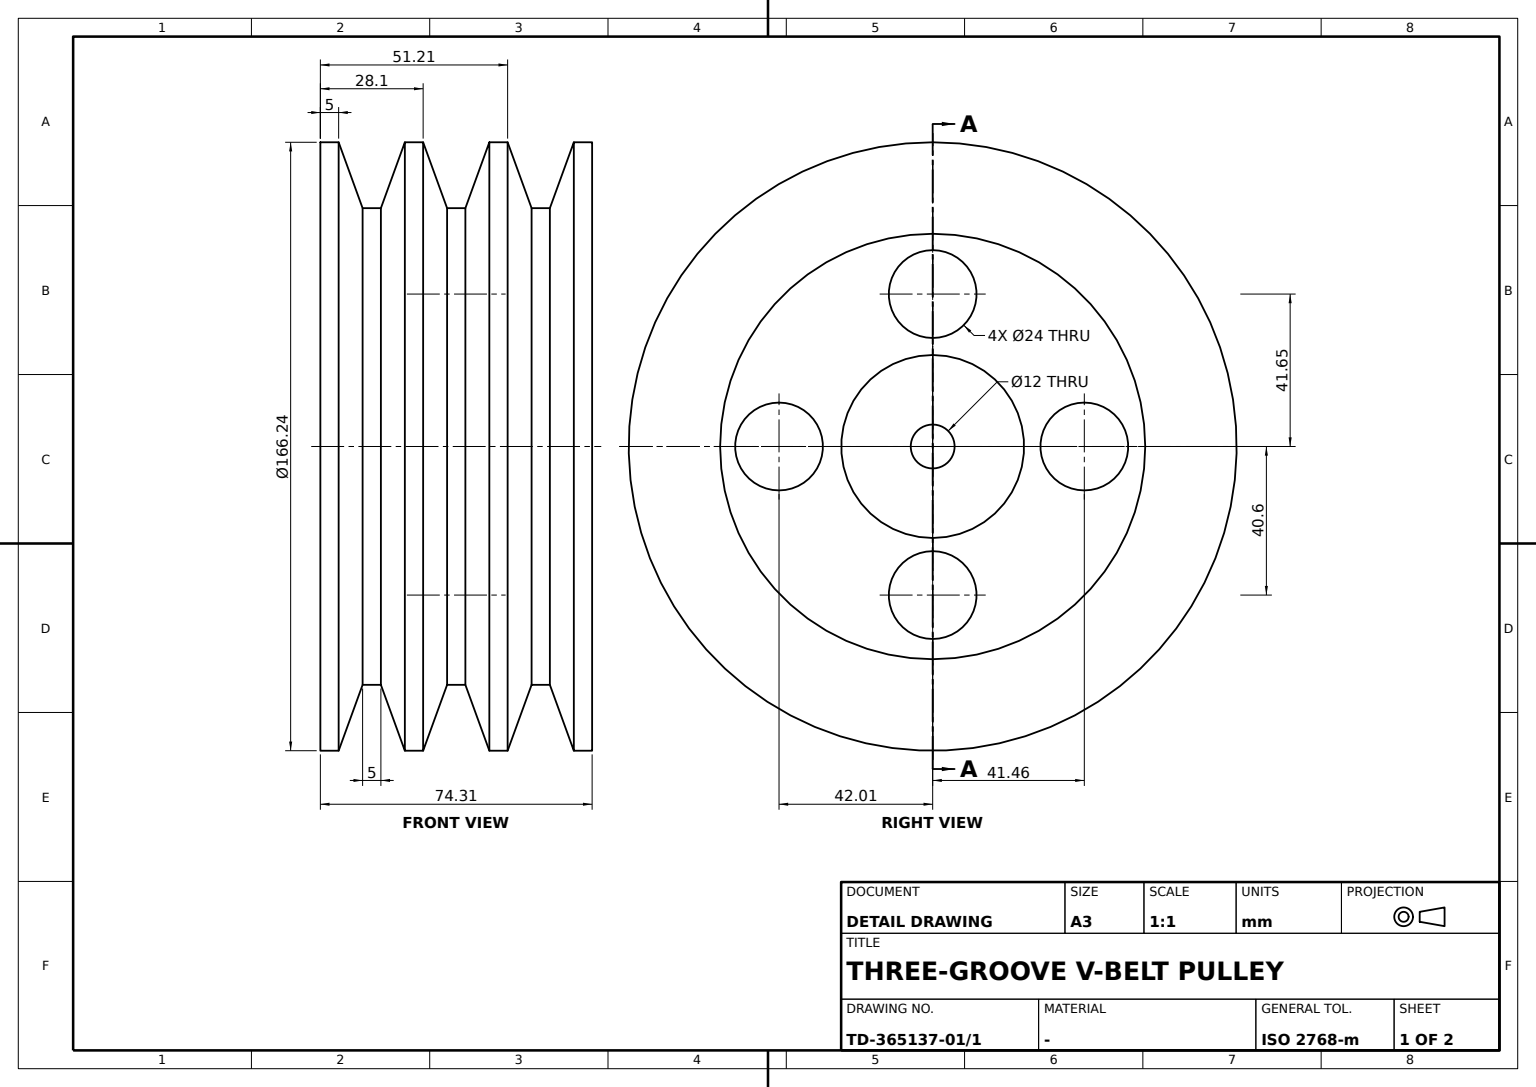
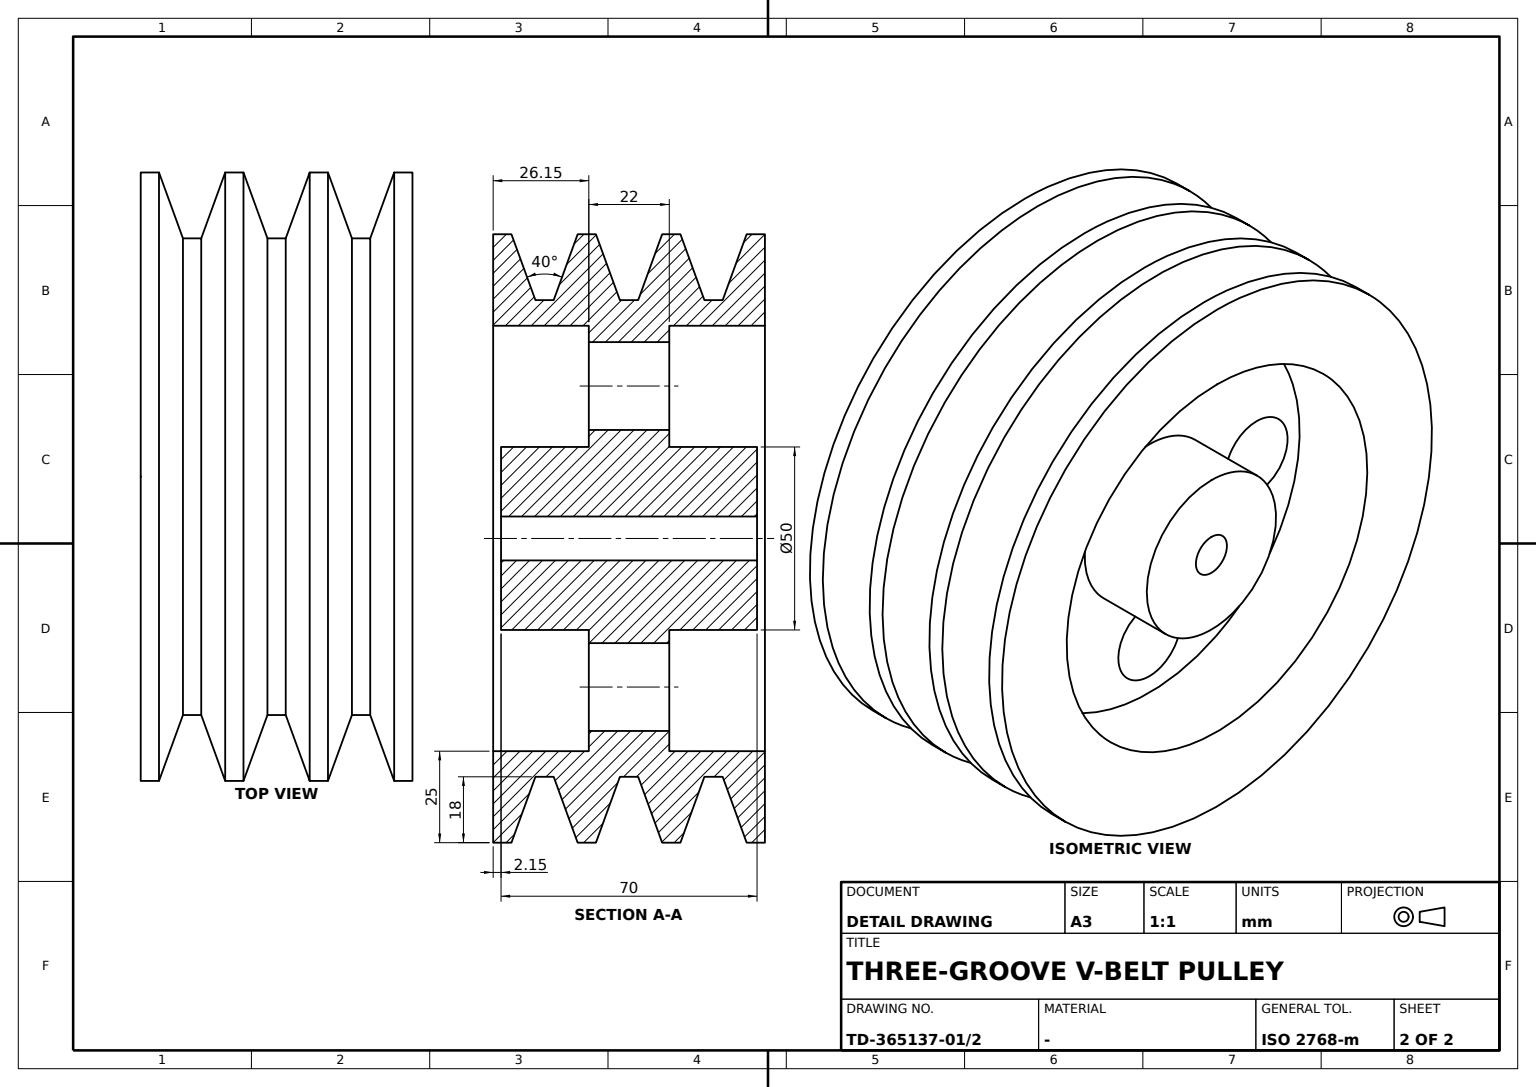
ISO-10303-21;
HEADER;
FILE_DESCRIPTION((''),'2;1');
FILE_NAME('','',(''),(''),'','','');
FILE_SCHEMA(('AUTOMOTIVE_DESIGN'));
ENDSEC;
DATA;
#1=APPLICATION_CONTEXT('');
#2=PRODUCT_CONTEXT('',#1,'mechanical');
#3=PRODUCT('','','',(#2));
#4=PRODUCT_DEFINITION_FORMATION('','',#3);
#5=PRODUCT_DEFINITION_CONTEXT('',#1,'design');
#6=PRODUCT_DEFINITION('','',#4,#5);
#7=PRODUCT_DEFINITION_SHAPE('','',#6);
#8=(LENGTH_UNIT()NAMED_UNIT(*)SI_UNIT(.MILLI.,.METRE.));
#9=(NAMED_UNIT(*)PLANE_ANGLE_UNIT()SI_UNIT($,.RADIAN.));
#10=(NAMED_UNIT(*)SI_UNIT($,.STERADIAN.)SOLID_ANGLE_UNIT());
#11=UNCERTAINTY_MEASURE_WITH_UNIT(LENGTH_MEASURE(0.005),#8,'distance_accuracy_value','');
#12=(GEOMETRIC_REPRESENTATION_CONTEXT(3)GLOBAL_UNCERTAINTY_ASSIGNED_CONTEXT((#11))GLOBAL_UNIT_ASSIGNED_CONTEXT((#8,#9,#10))REPRESENTATION_CONTEXT('',''));
#13=CARTESIAN_POINT('',(0.,-35.,6.));
#14=VERTEX_POINT('',#13);
#15=CARTESIAN_POINT('',(0.,-35.,0.));
#16=DIRECTION('',(0.,1.,0.));
#17=DIRECTION('',(0.,0.,1.));
#18=AXIS2_PLACEMENT_3D('',#15,#16,#17);
#19=CIRCLE('',#18,6.);
#20=EDGE_CURVE('',#14,#14,#19,.T.);
#21=ORIENTED_EDGE('',*,*,#20,.T.);
#22=EDGE_LOOP('',(#21));
#23=FACE_BOUND('',#22,.T.);
#24=CARTESIAN_POINT('',(0.,-35.,25.));
#25=VERTEX_POINT('',#24);
#26=CIRCLE('',#18,25.);
#27=EDGE_CURVE('',#25,#25,#26,.T.);
#28=ORIENTED_EDGE('',*,*,#27,.F.);
#29=EDGE_LOOP('',(#28));
#30=FACE_BOUND('',#29,.T.);
#31=DIRECTION('',(1.,0.,0.));
#32=AXIS2_PLACEMENT_3D('',#24,#16,#31);
#33=PLANE('',#32);
#34=ADVANCED_FACE('',(#23,#30),#33,.F.);
#35=CARTESIAN_POINT('',(0.,35.,25.));
#36=VERTEX_POINT('',#35);
#37=CARTESIAN_POINT('',(0.,35.,0.));
#38=AXIS2_PLACEMENT_3D('',#37,#16,#17);
#39=CIRCLE('',#38,25.);
#40=EDGE_CURVE('',#36,#36,#39,.T.);
#41=ORIENTED_EDGE('',*,*,#40,.T.);
#42=EDGE_LOOP('',(#41));
#43=FACE_BOUND('',#42,.T.);
#44=CARTESIAN_POINT('',(0.,35.,6.));
#45=VERTEX_POINT('',#44);
#46=CIRCLE('',#38,6.);
#47=EDGE_CURVE('',#45,#45,#46,.T.);
#48=ORIENTED_EDGE('',*,*,#47,.F.);
#49=EDGE_LOOP('',(#48));
#50=FACE_BOUND('',#49,.T.);
#51=AXIS2_PLACEMENT_3D('',#35,#16,#31);
#52=PLANE('',#51);
#53=ADVANCED_FACE('',(#43,#50),#52,.T.);
#54=CARTESIAN_POINT('',(0.,11.,-28.596905));
#55=VERTEX_POINT('',#54);
#56=CARTESIAN_POINT('',(0.,11.,-40.596905));
#57=AXIS2_PLACEMENT_3D('',#56,#16,#17);
#58=CIRCLE('',#57,12.);
#59=EDGE_CURVE('',#55,#55,#58,.T.);
#60=ORIENTED_EDGE('',*,*,#59,.T.);
#61=EDGE_LOOP('',(#60));
#62=FACE_BOUND('',#61,.T.);
#63=CARTESIAN_POINT('',(0.,-11.,-28.596905));
#64=VERTEX_POINT('',#63);
#65=CARTESIAN_POINT('',(0.,-11.,-40.596905));
#66=AXIS2_PLACEMENT_3D('',#65,#16,#17);
#67=CIRCLE('',#66,12.);
#68=EDGE_CURVE('',#64,#64,#67,.T.);
#69=ORIENTED_EDGE('',*,*,#68,.F.);
#70=EDGE_LOOP('',(#69));
#71=FACE_BOUND('',#70,.T.);
#72=CARTESIAN_POINT('',(0.,1.737196,-40.596905));
#73=DIRECTION('',(0.,-1.,0.));
#74=AXIS2_PLACEMENT_3D('',#72,#73,#31);
#75=CYLINDRICAL_SURFACE('',#74,12.);
#76=ADVANCED_FACE('',(#62,#71),#75,.F.);
#77=CARTESIAN_POINT('',(0.,-14.051464,83.121216));
#78=VERTEX_POINT('',#77);
#79=CARTESIAN_POINT('',(0.,-14.051464,0.));
#80=AXIS2_PLACEMENT_3D('',#79,#16,#17);
#81=CIRCLE('',#80,83.121216);
#82=EDGE_CURVE('',#78,#78,#81,.T.);
#83=ORIENTED_EDGE('',*,*,#82,.F.);
#84=EDGE_LOOP('',(#83));
#85=FACE_BOUND('',#84,.T.);
#86=CARTESIAN_POINT('',(0.,-20.602928,65.121216));
#87=VERTEX_POINT('',#86);
#88=CARTESIAN_POINT('',(0.,-20.602928,0.));
#89=AXIS2_PLACEMENT_3D('',#88,#16,#17);
#90=CIRCLE('',#89,65.121216);
#91=EDGE_CURVE('',#87,#87,#90,.T.);
#92=ORIENTED_EDGE('',*,*,#91,.T.);
#93=EDGE_LOOP('',(#92));
#94=FACE_BOUND('',#93,.T.);
#95=AXIS2_PLACEMENT_3D('',#88,#16,#31);
#96=CONICAL_SURFACE('',#95,65.121216129,1.221730476);
#97=ADVANCED_FACE('',(#85,#94),#96,.T.);
#98=CARTESIAN_POINT('',(-41.462753,-11.,12.));
#99=VERTEX_POINT('',#98);
#100=CARTESIAN_POINT('',(-41.462753,-11.,0.));
#101=AXIS2_PLACEMENT_3D('',#100,#16,#17);
#102=CIRCLE('',#101,12.);
#103=EDGE_CURVE('',#99,#99,#102,.T.);
#104=ORIENTED_EDGE('',*,*,#103,.T.);
#105=EDGE_LOOP('',(#104));
#106=FACE_BOUND('',#105,.T.);
#107=ORIENTED_EDGE('',*,*,#68,.T.);
#108=EDGE_LOOP('',(#107));
#109=FACE_BOUND('',#108,.T.);
#110=CARTESIAN_POINT('',(42.013649,-11.,12.));
#111=VERTEX_POINT('',#110);
#112=CARTESIAN_POINT('',(42.013649,-11.,0.));
#113=AXIS2_PLACEMENT_3D('',#112,#16,#17);
#114=CIRCLE('',#113,12.);
#115=EDGE_CURVE('',#111,#111,#114,.T.);
#116=ORIENTED_EDGE('',*,*,#115,.T.);
#117=EDGE_LOOP('',(#116));
#118=FACE_BOUND('',#117,.T.);
#119=CARTESIAN_POINT('',(0.,-11.,53.64854));
#120=VERTEX_POINT('',#119);
#121=CARTESIAN_POINT('',(0.,-11.,41.64854));
#122=AXIS2_PLACEMENT_3D('',#121,#16,#17);
#123=CIRCLE('',#122,12.);
#124=EDGE_CURVE('',#120,#120,#123,.T.);
#125=ORIENTED_EDGE('',*,*,#124,.T.);
#126=EDGE_LOOP('',(#125));
#127=FACE_BOUND('',#126,.T.);
#128=CARTESIAN_POINT('',(0.,-11.,25.));
#129=VERTEX_POINT('',#128);
#130=CARTESIAN_POINT('',(0.,-11.,0.));
#131=AXIS2_PLACEMENT_3D('',#130,#16,#17);
#132=CIRCLE('',#131,25.);
#133=EDGE_CURVE('',#129,#129,#132,.T.);
#134=ORIENTED_EDGE('',*,*,#133,.T.);
#135=EDGE_LOOP('',(#134));
#136=FACE_BOUND('',#135,.T.);
#137=CARTESIAN_POINT('',(0.,-11.,58.121216));
#138=VERTEX_POINT('',#137);
#139=CIRCLE('',#131,58.121216);
#140=EDGE_CURVE('',#138,#138,#139,.T.);
#141=ORIENTED_EDGE('',*,*,#140,.F.);
#142=EDGE_LOOP('',(#141));
#143=FACE_BOUND('',#142,.T.);
#144=AXIS2_PLACEMENT_3D('',#137,#16,#31);
#145=PLANE('',#144);
#146=ADVANCED_FACE('',(#106,#109,#118,#127,#136,#143),#145,.F.);
#147=CARTESIAN_POINT('',(0.,2.5,65.121216));
#148=VERTEX_POINT('',#147);
#149=CARTESIAN_POINT('',(0.,2.5,0.));
#150=AXIS2_PLACEMENT_3D('',#149,#16,#17);
#151=CIRCLE('',#150,65.121216);
#152=EDGE_CURVE('',#148,#148,#151,.T.);
#153=ORIENTED_EDGE('',*,*,#152,.T.);
#154=EDGE_LOOP('',(#153));
#155=FACE_BOUND('',#154,.T.);
#156=CARTESIAN_POINT('',(0.,9.051464,83.121216));
#157=VERTEX_POINT('',#156);
#158=CARTESIAN_POINT('',(0.,9.051464,0.));
#159=AXIS2_PLACEMENT_3D('',#158,#16,#17);
#160=CIRCLE('',#159,83.121216);
#161=EDGE_CURVE('',#157,#157,#160,.T.);
#162=ORIENTED_EDGE('',*,*,#161,.F.);
#163=EDGE_LOOP('',(#162));
#164=FACE_BOUND('',#163,.T.);
#165=AXIS2_PLACEMENT_3D('',#149,#16,#31);
#166=CONICAL_SURFACE('',#165,65.121216129,1.221730476);
#167=ADVANCED_FACE('',(#155,#164),#166,.T.);
#168=CARTESIAN_POINT('',(0.,11.,25.));
#169=VERTEX_POINT('',#168);
#170=CARTESIAN_POINT('',(0.,11.,0.));
#171=AXIS2_PLACEMENT_3D('',#170,#16,#17);
#172=CIRCLE('',#171,25.);
#173=EDGE_CURVE('',#169,#169,#172,.T.);
#174=ORIENTED_EDGE('',*,*,#173,.F.);
#175=EDGE_LOOP('',(#174));
#176=FACE_BOUND('',#175,.T.);
#177=ORIENTED_EDGE('',*,*,#59,.F.);
#178=EDGE_LOOP('',(#177));
#179=FACE_BOUND('',#178,.T.);
#180=CARTESIAN_POINT('',(0.,11.,58.121216));
#181=VERTEX_POINT('',#180);
#182=CIRCLE('',#171,58.121216);
#183=EDGE_CURVE('',#181,#181,#182,.T.);
#184=ORIENTED_EDGE('',*,*,#183,.T.);
#185=EDGE_LOOP('',(#184));
#186=FACE_BOUND('',#185,.T.);
#187=CARTESIAN_POINT('',(-41.462753,11.,12.));
#188=VERTEX_POINT('',#187);
#189=CARTESIAN_POINT('',(-41.462753,11.,0.));
#190=AXIS2_PLACEMENT_3D('',#189,#16,#17);
#191=CIRCLE('',#190,12.);
#192=EDGE_CURVE('',#188,#188,#191,.T.);
#193=ORIENTED_EDGE('',*,*,#192,.F.);
#194=EDGE_LOOP('',(#193));
#195=FACE_BOUND('',#194,.T.);
#196=CARTESIAN_POINT('',(0.,11.,53.64854));
#197=VERTEX_POINT('',#196);
#198=CARTESIAN_POINT('',(0.,11.,41.64854));
#199=AXIS2_PLACEMENT_3D('',#198,#16,#17);
#200=CIRCLE('',#199,12.);
#201=EDGE_CURVE('',#197,#197,#200,.T.);
#202=ORIENTED_EDGE('',*,*,#201,.F.);
#203=EDGE_LOOP('',(#202));
#204=FACE_BOUND('',#203,.T.);
#205=CARTESIAN_POINT('',(42.013649,11.,12.));
#206=VERTEX_POINT('',#205);
#207=CARTESIAN_POINT('',(42.013649,11.,0.));
#208=AXIS2_PLACEMENT_3D('',#207,#16,#17);
#209=CIRCLE('',#208,12.);
#210=EDGE_CURVE('',#206,#206,#209,.T.);
#211=ORIENTED_EDGE('',*,*,#210,.F.);
#212=EDGE_LOOP('',(#211));
#213=FACE_BOUND('',#212,.T.);
#214=AXIS2_PLACEMENT_3D('',#180,#16,#31);
#215=PLANE('',#214);
#216=ADVANCED_FACE('',(#176,#179,#186,#195,#204,#213),#215,.T.);
#217=CARTESIAN_POINT('',(0.,-9.051464,-83.121216));
#218=VERTEX_POINT('',#217);
#219=CARTESIAN_POINT('',(0.,-9.051464,0.));
#220=DIRECTION('',(0.,0.,-1.));
#221=AXIS2_PLACEMENT_3D('',#219,#73,#220);
#222=CIRCLE('',#221,83.121216);
#223=EDGE_CURVE('',#218,#218,#222,.F.);
#224=ORIENTED_EDGE('',*,*,#223,.F.);
#225=EDGE_LOOP('',(#224));
#226=FACE_BOUND('',#225,.T.);
#227=ORIENTED_EDGE('',*,*,#82,.T.);
#228=EDGE_LOOP('',(#227));
#229=FACE_BOUND('',#228,.T.);
#230=CARTESIAN_POINT('',(0.,0.,0.));
#231=AXIS2_PLACEMENT_3D('',#230,#16,#31);
#232=CYLINDRICAL_SURFACE('',#231,83.121216);
#233=ADVANCED_FACE('',(#226,#229),#232,.T.);
#234=ORIENTED_EDGE('',*,*,#152,.F.);
#235=EDGE_LOOP('',(#234));
#236=FACE_BOUND('',#235,.T.);
#237=CARTESIAN_POINT('',(0.,-2.5,-65.121216));
#238=VERTEX_POINT('',#237);
#239=CARTESIAN_POINT('',(0.,-2.5,0.));
#240=AXIS2_PLACEMENT_3D('',#239,#73,#220);
#241=CIRCLE('',#240,65.121216);
#242=EDGE_CURVE('',#238,#238,#241,.F.);
#243=ORIENTED_EDGE('',*,*,#242,.T.);
#244=EDGE_LOOP('',(#243));
#245=FACE_BOUND('',#244,.T.);
#246=CYLINDRICAL_SURFACE('',#231,65.121216);
#247=ADVANCED_FACE('',(#236,#245),#246,.T.);
#248=ORIENTED_EDGE('',*,*,#173,.T.);
#249=EDGE_LOOP('',(#248));
#250=FACE_BOUND('',#249,.T.);
#251=ORIENTED_EDGE('',*,*,#40,.F.);
#252=EDGE_LOOP('',(#251));
#253=FACE_BOUND('',#252,.T.);
#254=CYLINDRICAL_SURFACE('',#231,25.);
#255=ADVANCED_FACE('',(#250,#253),#254,.T.);
#256=ORIENTED_EDGE('',*,*,#201,.T.);
#257=EDGE_LOOP('',(#256));
#258=FACE_BOUND('',#257,.T.);
#259=ORIENTED_EDGE('',*,*,#124,.F.);
#260=EDGE_LOOP('',(#259));
#261=FACE_BOUND('',#260,.T.);
#262=CARTESIAN_POINT('',(0.,1.737196,41.64854));
#263=AXIS2_PLACEMENT_3D('',#262,#73,#31);
#264=CYLINDRICAL_SURFACE('',#263,12.);
#265=ADVANCED_FACE('',(#258,#261),#264,.F.);
#266=ORIENTED_EDGE('',*,*,#91,.F.);
#267=EDGE_LOOP('',(#266));
#268=FACE_BOUND('',#267,.T.);
#269=CARTESIAN_POINT('',(0.,-25.602928,-65.121216));
#270=VERTEX_POINT('',#269);
#271=CARTESIAN_POINT('',(0.,-25.602928,0.));
#272=AXIS2_PLACEMENT_3D('',#271,#73,#220);
#273=CIRCLE('',#272,65.121216);
#274=EDGE_CURVE('',#270,#270,#273,.F.);
#275=ORIENTED_EDGE('',*,*,#274,.T.);
#276=EDGE_LOOP('',(#275));
#277=FACE_BOUND('',#276,.T.);
#278=ADVANCED_FACE('',(#268,#277),#246,.T.);
#279=CARTESIAN_POINT('',(0.,-37.154393,83.121216));
#280=VERTEX_POINT('',#279);
#281=CARTESIAN_POINT('',(0.,-37.154393,0.));
#282=AXIS2_PLACEMENT_3D('',#281,#16,#17);
#283=CIRCLE('',#282,83.121216);
#284=EDGE_CURVE('',#280,#280,#283,.T.);
#285=ORIENTED_EDGE('',*,*,#284,.T.);
#286=EDGE_LOOP('',(#285));
#287=FACE_BOUND('',#286,.T.);
#288=CARTESIAN_POINT('',(0.,-32.154393,-83.121216));
#289=VERTEX_POINT('',#288);
#290=CARTESIAN_POINT('',(0.,-32.154393,0.));
#291=AXIS2_PLACEMENT_3D('',#290,#73,#220);
#292=CIRCLE('',#291,83.121216);
#293=EDGE_CURVE('',#289,#289,#292,.F.);
#294=ORIENTED_EDGE('',*,*,#293,.F.);
#295=EDGE_LOOP('',(#294));
#296=FACE_BOUND('',#295,.T.);
#297=ADVANCED_FACE('',(#287,#296),#232,.T.);
#298=CARTESIAN_POINT('',(0.,37.154393,83.121216));
#299=VERTEX_POINT('',#298);
#300=CARTESIAN_POINT('',(0.,37.154393,0.));
#301=AXIS2_PLACEMENT_3D('',#300,#16,#17);
#302=CIRCLE('',#301,83.121216);
#303=EDGE_CURVE('',#299,#299,#302,.T.);
#304=ORIENTED_EDGE('',*,*,#303,.F.);
#305=EDGE_LOOP('',(#304));
#306=FACE_BOUND('',#305,.T.);
#307=CARTESIAN_POINT('',(0.,32.154393,83.121216));
#308=VERTEX_POINT('',#307);
#309=CARTESIAN_POINT('',(0.,32.154393,0.));
#310=AXIS2_PLACEMENT_3D('',#309,#16,#17);
#311=CIRCLE('',#310,83.121216);
#312=EDGE_CURVE('',#308,#308,#311,.T.);
#313=ORIENTED_EDGE('',*,*,#312,.T.);
#314=EDGE_LOOP('',(#313));
#315=FACE_BOUND('',#314,.T.);
#316=ADVANCED_FACE('',(#306,#315),#232,.T.);
#317=ORIENTED_EDGE('',*,*,#312,.F.);
#318=EDGE_LOOP('',(#317));
#319=FACE_BOUND('',#318,.T.);
#320=CARTESIAN_POINT('',(0.,25.602928,65.121216));
#321=VERTEX_POINT('',#320);
#322=CARTESIAN_POINT('',(0.,25.602928,0.));
#323=AXIS2_PLACEMENT_3D('',#322,#16,#17);
#324=CIRCLE('',#323,65.121216);
#325=EDGE_CURVE('',#321,#321,#324,.T.);
#326=ORIENTED_EDGE('',*,*,#325,.T.);
#327=EDGE_LOOP('',(#326));
#328=FACE_BOUND('',#327,.T.);
#329=AXIS2_PLACEMENT_3D('',#322,#16,#31);
#330=CONICAL_SURFACE('',#329,65.121216129,1.221730476);
#331=ADVANCED_FACE('',(#319,#328),#330,.T.);
#332=ORIENTED_EDGE('',*,*,#274,.F.);
#333=EDGE_LOOP('',(#332));
#334=FACE_BOUND('',#333,.T.);
#335=ORIENTED_EDGE('',*,*,#293,.T.);
#336=EDGE_LOOP('',(#335));
#337=FACE_BOUND('',#336,.T.);
#338=AXIS2_PLACEMENT_3D('',#271,#73,#31);
#339=CONICAL_SURFACE('',#338,65.121216129,1.221730476);
#340=ADVANCED_FACE('',(#334,#337),#339,.T.);
#341=ORIENTED_EDGE('',*,*,#47,.T.);
#342=EDGE_LOOP('',(#341));
#343=FACE_BOUND('',#342,.T.);
#344=ORIENTED_EDGE('',*,*,#20,.F.);
#345=EDGE_LOOP('',(#344));
#346=FACE_BOUND('',#345,.T.);
#347=CYLINDRICAL_SURFACE('',#231,6.);
#348=ADVANCED_FACE('',(#343,#346),#347,.F.);
#349=ORIENTED_EDGE('',*,*,#192,.T.);
#350=EDGE_LOOP('',(#349));
#351=FACE_BOUND('',#350,.T.);
#352=ORIENTED_EDGE('',*,*,#103,.F.);
#353=EDGE_LOOP('',(#352));
#354=FACE_BOUND('',#353,.T.);
#355=CARTESIAN_POINT('',(-41.462753,1.737196,0.));
#356=AXIS2_PLACEMENT_3D('',#355,#73,#31);
#357=CYLINDRICAL_SURFACE('',#356,12.);
#358=ADVANCED_FACE('',(#351,#354),#357,.F.);
#359=CARTESIAN_POINT('',(0.,-37.154393,58.121216));
#360=VERTEX_POINT('',#359);
#361=CIRCLE('',#282,58.121216);
#362=EDGE_CURVE('',#360,#360,#361,.T.);
#363=ORIENTED_EDGE('',*,*,#362,.T.);
#364=EDGE_LOOP('',(#363));
#365=FACE_BOUND('',#364,.T.);
#366=ORIENTED_EDGE('',*,*,#284,.F.);
#367=EDGE_LOOP('',(#366));
#368=FACE_BOUND('',#367,.T.);
#369=AXIS2_PLACEMENT_3D('',#279,#16,#31);
#370=PLANE('',#369);
#371=ADVANCED_FACE('',(#365,#368),#370,.F.);
#372=CARTESIAN_POINT('',(0.,14.051464,-83.121216));
#373=VERTEX_POINT('',#372);
#374=CARTESIAN_POINT('',(0.,14.051464,0.));
#375=AXIS2_PLACEMENT_3D('',#374,#73,#220);
#376=CIRCLE('',#375,83.121216);
#377=EDGE_CURVE('',#373,#373,#376,.F.);
#378=ORIENTED_EDGE('',*,*,#377,.T.);
#379=EDGE_LOOP('',(#378));
#380=FACE_BOUND('',#379,.T.);
#381=CARTESIAN_POINT('',(0.,20.602928,-65.121216));
#382=VERTEX_POINT('',#381);
#383=CARTESIAN_POINT('',(0.,20.602928,0.));
#384=AXIS2_PLACEMENT_3D('',#383,#73,#220);
#385=CIRCLE('',#384,65.121216);
#386=EDGE_CURVE('',#382,#382,#385,.F.);
#387=ORIENTED_EDGE('',*,*,#386,.F.);
#388=EDGE_LOOP('',(#387));
#389=FACE_BOUND('',#388,.T.);
#390=AXIS2_PLACEMENT_3D('',#383,#73,#31);
#391=CONICAL_SURFACE('',#390,65.121216129,1.221730476);
#392=ADVANCED_FACE('',(#380,#389),#391,.T.);
#393=CARTESIAN_POINT('',(0.,37.154393,58.121216));
#394=VERTEX_POINT('',#393);
#395=CIRCLE('',#301,58.121216);
#396=EDGE_CURVE('',#394,#394,#395,.T.);
#397=ORIENTED_EDGE('',*,*,#396,.T.);
#398=EDGE_LOOP('',(#397));
#399=FACE_BOUND('',#398,.T.);
#400=ORIENTED_EDGE('',*,*,#183,.F.);
#401=EDGE_LOOP('',(#400));
#402=FACE_BOUND('',#401,.T.);
#403=CYLINDRICAL_SURFACE('',#231,58.121216);
#404=ADVANCED_FACE('',(#399,#402),#403,.F.);
#405=ORIENTED_EDGE('',*,*,#133,.F.);
#406=EDGE_LOOP('',(#405));
#407=FACE_BOUND('',#406,.T.);
#408=ORIENTED_EDGE('',*,*,#27,.T.);
#409=EDGE_LOOP('',(#408));
#410=FACE_BOUND('',#409,.T.);
#411=ADVANCED_FACE('',(#407,#410),#254,.T.);
#412=ORIENTED_EDGE('',*,*,#223,.T.);
#413=EDGE_LOOP('',(#412));
#414=FACE_BOUND('',#413,.T.);
#415=ORIENTED_EDGE('',*,*,#242,.F.);
#416=EDGE_LOOP('',(#415));
#417=FACE_BOUND('',#416,.T.);
#418=AXIS2_PLACEMENT_3D('',#239,#73,#31);
#419=CONICAL_SURFACE('',#418,65.121216129,1.221730476);
#420=ADVANCED_FACE('',(#414,#417),#419,.T.);
#421=ORIENTED_EDGE('',*,*,#386,.T.);
#422=EDGE_LOOP('',(#421));
#423=FACE_BOUND('',#422,.T.);
#424=ORIENTED_EDGE('',*,*,#325,.F.);
#425=EDGE_LOOP('',(#424));
#426=FACE_BOUND('',#425,.T.);
#427=ADVANCED_FACE('',(#423,#426),#246,.T.);
#428=ORIENTED_EDGE('',*,*,#377,.F.);
#429=EDGE_LOOP('',(#428));
#430=FACE_BOUND('',#429,.T.);
#431=ORIENTED_EDGE('',*,*,#161,.T.);
#432=EDGE_LOOP('',(#431));
#433=FACE_BOUND('',#432,.T.);
#434=ADVANCED_FACE('',(#430,#433),#232,.T.);
#435=ORIENTED_EDGE('',*,*,#362,.F.);
#436=EDGE_LOOP('',(#435));
#437=FACE_BOUND('',#436,.T.);
#438=ORIENTED_EDGE('',*,*,#140,.T.);
#439=EDGE_LOOP('',(#438));
#440=FACE_BOUND('',#439,.T.);
#441=ADVANCED_FACE('',(#437,#440),#403,.F.);
#442=ORIENTED_EDGE('',*,*,#210,.T.);
#443=EDGE_LOOP('',(#442));
#444=FACE_BOUND('',#443,.T.);
#445=ORIENTED_EDGE('',*,*,#115,.F.);
#446=EDGE_LOOP('',(#445));
#447=FACE_BOUND('',#446,.T.);
#448=CARTESIAN_POINT('',(42.013649,1.737196,0.));
#449=AXIS2_PLACEMENT_3D('',#448,#73,#31);
#450=CYLINDRICAL_SURFACE('',#449,12.);
#451=ADVANCED_FACE('',(#444,#447),#450,.F.);
#452=ORIENTED_EDGE('',*,*,#396,.F.);
#453=EDGE_LOOP('',(#452));
#454=FACE_BOUND('',#453,.T.);
#455=ORIENTED_EDGE('',*,*,#303,.T.);
#456=EDGE_LOOP('',(#455));
#457=FACE_BOUND('',#456,.T.);
#458=AXIS2_PLACEMENT_3D('',#298,#16,#31);
#459=PLANE('',#458);
#460=ADVANCED_FACE('',(#454,#457),#459,.T.);
#461=CLOSED_SHELL('',(#34,#53,#76,#97,#146,#167,#216,#233,#247,#255,#265,#278,#297,#316,#331,#340,#348,#358,#371,#392,#404,#411,#420,#427,#434,#441,#451,#460));
#462=MANIFOLD_SOLID_BREP('',#461);
#463=ADVANCED_BREP_SHAPE_REPRESENTATION('',(#462),#12);
#464=SHAPE_DEFINITION_REPRESENTATION(#7,#463);
ENDSEC;
END-ISO-10303-21;
